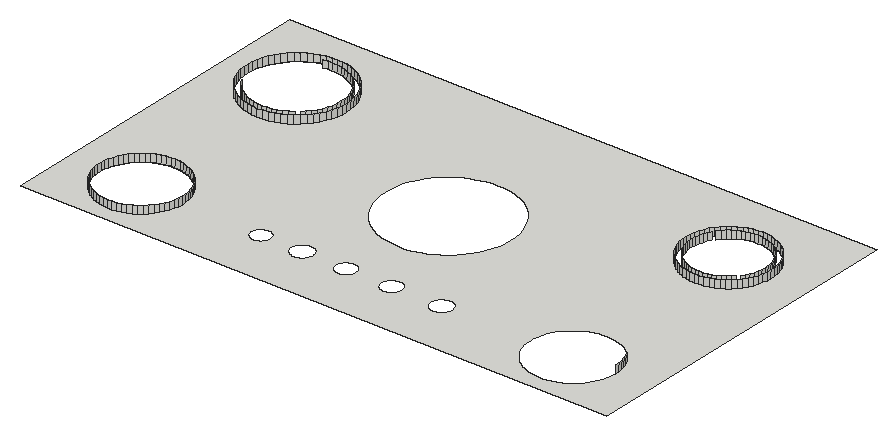
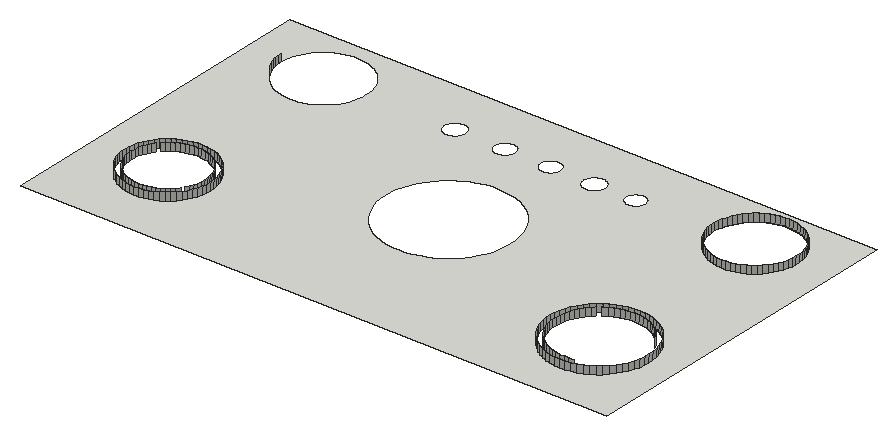
# SketchUp Ruby script. Lengths in inches.
U = 1.inch
M = Sketchup.active_model
def pt(a) = Geom::Point3d.new(a.map { |v| v * U })
def face(e, loops, mat)
  f = e.add_face(loops[0].map { |a| pt(a) })
  loops[1..].each { |l| e.add_face(l.map { |a| pt(a) }).erase! }
  f.material = f.back_material = mat if mat
  f
end
# faces: each face lists its corners as indices into pts; further lists are holes
def faces(e, pts, list, mat = nil) = list.each { |f| face(e, (f[0].is_a?(Array) ? f : [f]).map { |l| l.map { |i| pts[i] } }, mat) }
# xy, xz, yz: faces in a plane at the given z, y or x. An outline is a flat list of corners, or four numbers for a rectangle; further outlines are holes
def ring(l) = l.size == 4 ? [[l[0], l[1]], [l[2], l[1]], [l[2], l[3]], [l[0], l[3]]] : l.each_slice(2).to_a
def flat(e, list, mat, &to3) = list.each { |f| face(e, (f[0].is_a?(Array) ? f : [f]).map { |l| ring(l).map { |u, v| to3.(u, v) } }, mat) }
def xy(e, z, list, mat = nil) = flat(e, list, mat) { |x, y| [x, y, z] }
def xz(e, y, list, mat = nil) = flat(e, list, mat) { |x, z| [x, y, z] }
def yz(e, x, list, mat = nil) = flat(e, list, mat) { |y, z| [x, y, z] }
def lines(e, pts, list) = list.each { |a, b| e.add_line(pt(pts[a]), pt(pts[b])) }
# prism: a flat outline (further loops are holes) pulled along v
def prism(e, loops, v, mat = nil)
  f = face(e, loops, mat); d = Geom::Vector3d.new(v.map { |x| x * U })
  f.pushpull(f.normal.samedirection?(d) ? d.length : -d.length)
end
def box(e, o, s, mat = nil) = prism(e, [[o, [o[0] + s[0], o[1], o[2]], [o[0] + s[0], o[1] + s[1], o[2]], [o[0], o[1] + s[1], o[2]]]], [0, 0, s[2]], mat)
def at(x, y, z, deg = 0) = Geom::Transformation.translation(pt([x, y, z])) * Geom::Transformation.rotation(ORIGIN, Z_AXIS, deg.degrees)
def axes(o, x, y, z) = Geom::Transformation.new([*x, 0, *y, 0, *z, 0, *pt(o).to_a, 1])
def part(name) = M.definitions.add(name)
# library, detail: a bought-in or finely detailed component or shape, given as its bounding box
def library(name, o, s) = part(name).tap { |d| box(d.entities, o, s) }
def detail(e, o, s) = box(e.add_group.entities, o, s)
def put(e, d, t, mat = nil) = e.add_instance(d, t).tap { |i| i.material = mat if mat }
def group(e, t, mat = nil) = e.add_group.tap { |g| g.transformation = t; g.material = mat if mat }.entities
root = M.entities
xy(root,253.1875,[[[597.55,622.78,883.3,786.9],[739.6875,675.19,736.49,675.36,733.32,675.86,730.22,676.69,727.23,677.84,724.375,679.29,721.6875,681.04,719.19,683.06,716.93,685.32,714.91,687.82,713.16,690.5,711.71,693.36,710.5625,696.35,709.73,699.45,709.23,702.61,709.0625,705.82,709.23,709.02,709.73,712.18,710.5625,715.28,711.71,718.27,713.16,721.13,714.91,723.82,716.93,726.31,719.19,728.57,721.6875,730.59,724.375,732.34,727.23,733.79,730.22,734.94,733.32,735.77,736.49,736.27,739.6875,736.44,742.89,736.27,746.05,735.77,749.15,734.94,752.14,733.79,755,732.34,757.6875,730.59,760.18,728.57,762.45,726.31,764.46,723.82,766.21,721.13,767.66,718.27,768.8125,715.28,769.64,712.18,770.14,709.02,770.3125,705.82,770.14,702.61,769.64,699.45,768.8125,696.35,767.66,693.36,766.21,690.5,764.46,687.82,762.45,685.32,760.18,683.06,757.6875,681.04,755,679.29,752.14,677.84,749.15,676.69,746.05,675.86,742.89,675.36],[634.71,720.65,632.18,720.78,629.67,721.18,627.22,721.84,624.85,722.74,622.58,723.9,620.46,725.28,618.48,726.875,616.6875,728.67,615.09,730.64,613.71,732.77,612.56,735.03,611.65,737.4,610.99,739.86,610.59,742.36,610.46,744.9,610.59,747.43,610.99,749.94,611.65,752.39,612.56,754.76,613.71,757.02,615.09,759.15,616.6875,761.125,618.48,762.92,620.46,764.52,622.58,765.9,624.85,767.05,627.22,767.96,629.67,768.62,632.18,769.02,634.71,769.15,637.24,769.02,639.75,768.62,642.2,767.96,644.57,767.05,646.83,765.9,648.96,764.52,650.9375,762.92,652.73,761.125,654.33,759.15,655.71,757.02,656.86,754.76,657.77,752.39,658.43,749.94,658.83,747.43,658.96,744.9,658.83,742.36,658.43,739.86,657.77,737.4,656.86,735.03,655.71,732.77,654.33,730.64,652.73,728.67,650.9375,726.875,648.96,725.28,646.83,723.9,644.57,722.74,642.2,721.84,639.75,721.18,637.24,720.78],[844.95,724.15,842.78,724.26,840.64,724.6,838.54,725.16,836.51,725.94,834.58,726.93,832.76,728.11,831.07,729.48,829.53,731.01,828.16,732.7,826.98,734.52,826,736.46,825.22,738.49,824.66,740.58,824.32,742.73,824.2,744.9,824.32,747.07,824.66,749.21,825.22,751.31,826,753.34,826.98,755.27,828.16,757.09,829.53,758.78,831.07,760.32,832.76,761.69,834.58,762.87,836.51,763.85,838.54,764.63,840.64,765.19,842.78,765.53,844.95,765.65,847.12,765.53,849.27,765.19,851.36,764.63,853.39,763.85,855.33,762.87,857.15,761.69,858.84,760.32,860.37,758.78,861.74,757.09,862.92,755.27,863.91,753.34,864.6875,751.31,865.25,749.21,865.59,747.07,865.7,744.9,865.59,742.73,865.25,740.58,864.6875,738.49,863.91,736.46,862.92,734.52,861.74,732.7,860.37,731.01,858.84,729.48,857.15,728.11,855.33,726.93,853.39,725.94,851.36,725.16,849.27,724.6,847.12,724.26],[844.95,629.31,842.78,629.42,840.64,629.76,838.54,630.32,836.51,631.1,834.58,632.09,832.76,633.27,831.07,634.64,829.53,636.17,828.16,637.86,826.98,639.68,826,641.62,825.22,643.65,824.66,645.74,824.32,647.89,824.2,650.06,824.32,652.23,824.66,654.375,825.22,656.47,826,658.5,826.98,660.43,828.16,662.26,829.53,663.94,831.07,665.48,832.76,666.85,834.58,668.03,836.51,669.02,838.54,669.79,840.64,670.36,842.78,670.7,844.95,670.81,847.12,670.7,849.27,670.36,851.36,669.79,853.39,669.02,855.33,668.03,857.15,666.85,858.84,665.48,860.37,663.94,861.74,662.26,862.92,660.43,863.91,658.5,864.6875,656.47,865.25,654.375,865.59,652.23,865.7,650.06,865.59,647.89,865.25,645.74,864.6875,643.65,863.91,641.62,862.92,639.68,861.74,637.86,860.37,636.17,858.84,634.64,857.15,633.27,855.33,632.09,853.39,631.1,851.36,630.32,849.27,629.76,847.12,629.42],[634.4,629.8125,632.28,629.96,630.19,630.32,628.15,630.9,626.1875,631.69,624.3125,632.68,622.55,633.86,620.93,635.22,619.45,636.74,618.14,638.41,617.02,640.21,616.08,642.11,615.36,644.1,614.84,646.16,614.54,648.26,614.46,650.375,614.61,652.49,614.97,654.58,615.55,656.61,616.34,658.58,617.33,660.45,618.51,662.21,619.875,663.84,621.4,665.32,623.0625,666.625,624.86,667.75,626.76,668.68,628.75,669.41,630.81,669.93,632.91,670.23,635.02,670.31,637.14,670.16,639.23,669.8,641.27,669.22,643.23,668.43,645.11,667.4375,646.87,666.25,648.49,664.9,649.97,663.375,651.28,661.71,652.4,659.91,653.33,658.01,654.0625,656.02,654.58,653.96,654.88,651.86,654.96,649.74,654.8125,647.63,654.45,645.54,653.87,643.5,653.08,641.54,652.09,639.66,650.91,637.9,649.55,636.28,648.02,634.8,646.36,633.49,644.5625,632.37,642.66,631.43,640.67,630.71,638.61,630.1875,636.51,629.89],[713.34,644.32,712.77,644.35,712.21,644.4375,711.66,644.58,711.125,644.79,710.62,645.05,710.14,645.36,709.7,645.71,709.3,646.12,708.9375,646.56,708.63,647.04,708.37,647.54,708.17,648.07,708.02,648.625,707.93,649.1875,707.9,649.75,707.93,650.32,708.02,650.89,708.17,651.43,708.37,651.97,708.63,652.47,708.9375,652.95,709.3,653.39,709.7,653.8,710.14,654.15,710.62,654.46,711.125,654.72,711.66,654.93,712.21,655.07,712.77,655.16,713.34,655.19,713.91,655.16,714.47,655.07,715.02,654.93,715.55,654.72,716.06,654.46,716.53,654.15,716.98,653.8,717.38,653.39,717.74,652.95,718.05,652.47,718.31,651.97,718.51,651.43,718.66,650.89,718.75,650.32,718.78,649.75,718.75,649.1875,718.66,648.625,718.51,648.07,718.31,647.54,718.05,647.04,717.74,646.56,717.38,646.12,716.98,645.71,716.53,645.36,716.06,645.05,715.55,644.79,715.02,644.58,714.47,644.4375,713.91,644.35],[781.2,644.44,780.65,644.47,780.1,644.56,779.5625,644.7,779.04,644.9,778.55,645.15,778.08,645.46,777.65,645.81,777.26,646.2,776.91,646.63,776.6,647.1,776.35,647.59,776.15,648.11,776.01,648.65,775.92,649.2,775.89,649.75,775.92,650.31,776.01,650.86,776.15,651.4,776.35,651.92,776.6,652.41,776.91,652.88,777.26,653.31,777.65,653.7,778.08,654.05,778.55,654.36,779.04,654.61,779.5625,654.81,780.1,654.95,780.65,655.04,781.2,655.07,781.76,655.04,782.31,654.95,782.85,654.81,783.36,654.61,783.86,654.36,784.33,654.05,784.76,653.7,785.15,653.31,785.5,652.88,785.8,652.41,786.06,651.92,786.26,651.4,786.4,650.86,786.49,650.31,786.52,649.75,786.49,649.2,786.4,648.65,786.26,648.11,786.06,647.59,785.8,647.1,785.5,646.63,785.15,646.2,784.76,645.81,784.33,645.46,783.86,645.15,783.36,644.9,782.85,644.7,782.31,644.56,781.76,644.47],[756.84,644.69,756.3125,644.72,755.79,644.8,755.28,644.94,754.78,645.13,754.31,645.37,753.86,645.66,753.45,645.99,753.08,646.37,752.74,646.78,752.46,647.22,752.21,647.7,752.02,648.19,751.89,648.7,751.8,649.23,751.78,649.75,751.8,650.28,751.89,650.81,752.02,651.32,752.21,651.8125,752.46,652.29,752.74,652.73,753.08,653.14,753.45,653.52,753.86,653.85,754.31,654.14,754.78,654.38,755.28,654.57,755.79,654.71,756.3125,654.79,756.84,654.82,757.37,654.79,757.89,654.71,758.4,654.57,758.9,654.38,759.37,654.14,759.82,653.85,760.23,653.52,760.6,653.14,760.94,652.73,761.22,652.29,761.46,651.8125,761.65,651.32,761.79,650.81,761.875,650.28,761.9,649.75,761.875,649.23,761.79,648.7,761.65,648.19,761.46,647.7,761.22,647.22,760.94,646.78,760.6,646.37,760.23,645.99,759.82,645.66,759.37,645.37,758.9,645.13,758.4,644.94,757.89,644.8,757.37,644.72],[734.71,644.78,734.19,644.81,733.68,644.89,733.18,645.03,732.69,645.21,732.23,645.45,731.79,645.73,731.39,646.06,731.02,646.43,730.69,646.83,730.41,647.27,730.17,647.73,729.98,648.22,729.85,648.72,729.77,649.23,729.74,649.75,729.77,650.27,729.85,650.79,729.98,651.29,730.17,651.78,730.41,652.24,730.69,652.68,731.02,653.08,731.39,653.45,731.79,653.78,732.23,654.0625,732.69,654.3,733.18,654.48,733.68,654.62,734.19,654.7,734.71,654.73,735.23,654.7,735.75,654.62,736.25,654.48,736.74,654.3,737.2,654.0625,737.64,653.78,738.04,653.45,738.41,653.08,738.74,652.68,739.02,652.24,739.26,651.78,739.44,651.29,739.58,650.79,739.66,650.27,739.6875,649.75,739.66,649.23,739.58,648.72,739.44,648.22,739.26,647.73,739.02,647.27,738.74,646.83,738.41,646.43,738.04,646.06,737.64,645.73,737.2,645.45,736.74,645.21,736.25,645.03,735.75,644.89,735.23,644.81],[693.15,644.94,692.64,644.97,692.14,645.05,691.66,645.18,691.1875,645.36,690.74,645.59,690.32,645.86,689.93,646.18,689.57,646.53,689.25,646.93,688.98,647.35,688.75,647.8,688.57,648.27,688.4375,648.75,688.36,649.25,688.33,649.75,688.36,650.26,688.4375,650.76,688.57,651.24,688.75,651.71,688.98,652.16,689.25,652.58,689.57,652.97,689.93,653.33,690.32,653.65,690.74,653.92,691.1875,654.15,691.66,654.33,692.14,654.46,692.64,654.54,693.15,654.57,693.65,654.54,694.15,654.46,694.63,654.33,695.1,654.15,695.55,653.92,695.97,653.65,696.37,653.33,696.72,652.97,697.04,652.58,697.3125,652.16,697.54,651.71,697.72,651.24,697.85,650.76,697.93,650.26,697.96,649.75,697.93,649.25,697.85,648.75,697.72,648.27,697.54,647.8,697.3125,647.35,697.04,646.93,696.72,646.53,696.37,646.18,695.97,645.86,695.55,645.59,695.1,645.36,694.63,645.18,694.15,645.05,693.65,644.97]]])
p = [[632.28,629.96,253.1875],[634.4,629.8125,253.1875],[634.4,629.8125,256.875],[632.28,629.96,256.875],[636.51,629.89,253.1875],[636.51,629.89,256.875],
  [638.61,630.1875,253.1875],[638.61,630.1875,256.875],[630.19,630.32,253.1875],[630.19,630.32,256.875],[640.67,630.71,253.1875],[640.67,630.71,256.875],
  [628.15,630.9,253.1875],[628.15,630.9,256.875],[642.66,631.43,253.1875],[642.66,631.43,256.875],[626.1875,631.69,253.1875],[626.1875,631.69,256.875],
  [644.5625,632.37,253.1875],[644.5625,632.37,256.875],[624.3125,632.68,253.1875],[624.3125,632.68,256.875],[646.36,633.49,253.1875],[646.36,633.49,256.875],
  [622.55,633.86,253.1875],[622.55,633.86,256.875],[648.02,634.8,253.1875],[648.02,634.8,256.875],[620.93,635.22,253.1875],[620.93,635.22,256.875],
  [649.55,636.28,253.1875],[649.55,636.28,256.875],[619.45,636.74,253.1875],[619.45,636.74,256.875],[650.91,637.9,253.1875],[650.91,637.9,256.875],
  [618.14,638.41,253.1875],[618.14,638.41,256.875],[652.09,639.66,253.1875],[652.09,639.66,256.875],[617.02,640.21,253.1875],[617.02,640.21,256.875],
  [653.08,641.54,253.1875],[653.08,641.54,256.875],[616.08,642.11,253.1875],[616.08,642.11,256.875],[653.87,643.5,253.1875],[653.87,643.5,256.875],
  [615.36,644.1,253.1875],[615.36,644.1,256.875],[654.45,645.54,253.1875],[654.45,645.54,256.875],[614.84,646.16,253.1875],[614.84,646.16,256.875],
  [654.8125,647.63,253.1875],[654.8125,647.63,256.875],[614.54,648.26,253.1875],[614.54,648.26,256.875],[654.96,649.74,253.1875],[654.96,649.74,256.875],
  [614.46,650.375,253.1875],[614.46,650.375,256.875],[654.88,651.86,253.1875],[654.88,651.86,256.875],[865.7,650.06,253.1875],[865.59,652.23,253.1875],
  [865.59,652.23,256.875],[865.7,650.06,256.875],[614.61,652.49,253.1875],[614.61,652.49,256.875],[654.58,653.96,253.1875],[654.58,653.96,256.875],
  [865.25,654.375,253.1875],[865.25,654.375,256.875],[614.97,654.58,253.1875],[614.97,654.58,256.875],[654.0625,656.02,253.1875],[654.0625,656.02,256.875],
  [864.6875,656.47,253.1875],[864.6875,656.47,256.875],[615.55,656.61,253.1875],[615.55,656.61,256.875],[653.33,658.01,253.1875],[653.33,658.01,256.875],
  [863.91,658.5,253.1875],[863.91,658.5,256.875],[616.34,658.58,253.1875],[616.34,658.58,256.875],[652.4,659.91,253.1875],[652.4,659.91,256.875],
  [862.92,660.43,253.1875],[862.92,660.43,256.875],[617.33,660.45,253.1875],[617.33,660.45,256.875],[651.28,661.71,253.1875],[651.28,661.71,256.875],
  [618.51,662.21,253.1875],[618.51,662.21,256.875],[649.97,663.375,253.1875],[649.97,663.375,256.875],[619.875,663.84,253.1875],[619.875,663.84,256.875],
  [648.49,664.9,253.1875],[648.49,664.9,256.875],[621.4,665.32,253.1875],[621.4,665.32,256.875],[646.87,666.25,253.1875],[646.87,666.25,256.875],
  [623.0625,666.625,253.1875],[623.0625,666.625,256.875],[645.11,667.4375,253.1875],[645.11,667.4375,256.875],[624.86,667.75,253.1875],[624.86,667.75,256.875],
  [643.23,668.43,253.1875],[643.23,668.43,256.875],[626.76,668.68,253.1875],[626.76,668.68,256.875],[641.27,669.22,253.1875],[641.27,669.22,256.875],
  [628.75,669.41,253.1875],[628.75,669.41,256.875],[639.23,669.8,253.1875],[639.23,669.8,256.875],[630.81,669.93,253.1875],[630.81,669.93,256.875],
  [637.14,670.16,253.1875],[637.14,670.16,256.875],[632.91,670.23,253.1875],[632.91,670.23,256.875],[635.02,670.31,253.1875],[635.02,670.31,256.875],
  [632.18,720.78,253.1875],[634.71,720.65,253.1875],[634.71,720.65,256.875],[632.18,720.78,256.875],[637.24,720.78,253.1875],[637.24,720.78,256.875],
  [629.67,721.18,253.1875],[629.67,721.18,256.875],[639.75,721.18,253.1875],[639.75,721.18,256.875],[627.22,721.84,253.1875],[627.22,721.84,256.875],
  [642.2,721.84,253.1875],[642.2,721.84,256.875],[624.85,722.74,253.1875],[624.85,722.74,256.875],[644.57,722.74,253.1875],[644.57,722.74,256.875],
  [622.58,723.9,253.1875],[622.58,723.9,256.875],[646.83,723.9,253.1875],[646.83,723.9,256.875],[634.71,723.48,253.1875],[632.47,723.59,253.1875],
  [632.47,723.59,256.875],[634.71,723.48,256.875],[636.95,723.59,253.1875],[636.95,723.59,256.875],[630.26,723.94,253.1875],[630.26,723.94,256.875],
  [639.16,723.94,253.1875],[639.16,723.94,256.875],[620.46,725.28,253.1875],[620.46,725.28,256.875],[628.09,724.53,253.1875],[628.09,724.53,256.875],
  [641.33,724.53,253.1875],[641.33,724.53,256.875],[648.96,725.28,253.1875],[648.96,725.28,256.875],[842.78,724.26,253.1875],[844.95,724.15,253.1875],
  [844.95,724.15,256.875],[842.78,724.26,256.875],[847.12,724.26,253.1875],[847.12,724.26,256.875],[840.64,724.6,253.1875],[840.64,724.6,256.875],
  [849.27,724.6,253.1875],[849.27,724.6,256.875],[626,725.33,253.1875],[626,725.33,256.875],[643.42,725.33,253.1875],[643.42,725.33,256.875],
  [838.54,725.16,253.1875],[838.54,725.16,256.875],[851.36,725.16,253.1875],[851.36,725.16,256.875],[836.51,725.94,253.1875],[836.51,725.94,256.875],
  [853.39,725.94,253.1875],[853.39,725.94,256.875],[618.48,726.875,253.1875],[618.48,726.875,256.875],[624,726.35,253.1875],[624,726.35,256.875],
  [645.42,726.35,253.1875],[645.42,726.35,256.875],[650.9375,726.875,253.1875],[650.9375,726.875,256.875],[834.58,726.93,253.1875],[834.58,726.93,256.875],
  [855.33,726.93,253.1875],[855.33,726.93,256.875],[622.12,727.57,253.1875],[622.12,727.57,256.875],[647.3,727.57,253.1875],[647.3,727.57,256.875],
  [647.3,727.57,255.1875],[616.6875,728.67,253.1875],[616.6875,728.67,256.875],[652.73,728.67,253.1875],[652.73,728.67,256.875],[832.76,728.11,253.1875],
  [832.76,728.11,256.875],[857.15,728.11,253.1875],[857.15,728.11,256.875],[844.95,726.98,253.1875],[843.08,727.07,253.1875],[843.08,727.07,256.875],
  [844.95,726.98,256.875],[846.82,727.07,253.1875],[846.82,727.07,256.875],[841.23,727.37,253.1875],[841.23,727.37,256.875],[848.68,727.37,253.1875],
  [848.68,727.37,256.875],[839.41,727.85,253.1875],[839.41,727.85,256.875],[850.49,727.85,253.1875],[850.49,727.85,256.875],[620.375,728.98,253.1875],
  [620.375,728.98,256.875],[837.66,728.53,253.1875],[837.66,728.53,256.875],[852.24,728.53,253.1875],[852.24,728.53,256.875],[831.07,729.48,253.1875],
  [831.07,729.48,256.875],[858.84,729.48,253.1875],[858.84,729.48,256.875],[835.99,729.38,253.1875],[835.99,729.38,256.875],[853.91,729.38,253.1875],
  [853.91,729.38,256.875],[615.09,730.64,253.1875],[615.09,730.64,256.875],[654.33,730.64,253.1875],[654.33,730.64,256.875],[619.69,729.66,253.1875],
  [619.69,729.66,255.1875],[618.79,730.5625,255.1875],[618.79,730.5625,256.875],[650.63,730.5625,253.1875],[649.04,728.98,253.1875],[649.04,728.98,255.1875],
  [649.04,728.98,256.875],[650.63,730.5625,256.875],[834.42,730.4,253.1875],[834.42,730.4,254.5],[834.42,730.4,256.875],[855.49,730.4,253.1875],
  [855.49,730.4,256.875],[829.53,731.01,253.1875],[829.53,731.01,256.875],[860.37,731.01,253.1875],[860.37,731.01,256.875],[856.94,731.58,253.1875],
  [856.94,731.58,256.875],[613.71,732.77,253.1875],[613.71,732.77,256.875],[618.09,731.4375,255.1875],[618.09,731.4375,253.1875],[617.38,732.31,253.1875],
  [617.38,732.31,256.875],[652.04,732.31,253.1875],[652.04,732.31,256.875],[655.71,732.77,253.1875],[655.71,732.77,256.875],[828.16,732.7,253.1875],
  [828.16,732.7,256.875],[861.74,732.7,253.1875],[861.74,732.7,256.875],[832.96,731.58,253.1875],[831.63,732.91,253.1875],[831.63,732.91,256.875],
  [832.96,731.58,256.875],[832.96,731.58,254.5],[858.27,732.91,253.1875],[858.27,732.91,256.875],[858.27,732.91,254.5],[616.16,734.1875,253.1875],
  [616.16,734.1875,256.875],[653.26,734.1875,253.1875],[653.26,734.1875,256.875],[826.98,734.52,253.1875],[826.98,734.52,256.875],[862.92,734.52,253.1875],
  [862.92,734.52,256.875],[612.56,735.03,253.1875],[612.56,735.03,256.875],[656.86,735.03,253.1875],[656.86,735.03,256.875],[830.45,734.36,253.1875],
  [830.45,734.36,256.875],[654.28,736.19,253.1875],[654.28,736.19,256.875],[829.43,735.9375,253.1875],[829.43,735.9375,256.875],[860.47,735.9375,253.1875],
  [859.45,734.36,253.1875],[859.45,734.36,254.5],[859.45,734.36,256.875],[860.47,735.9375,256.875],[826,736.46,253.1875],[826,736.46,256.875],
  [863.91,736.46,253.1875],[863.91,736.46,256.875],[611.65,737.4,253.1875],[611.65,737.4,256.875],[657.77,737.4,253.1875],[657.77,737.4,256.875],
  [828.58,737.61,253.1875],[828.58,737.61,256.875],[861.32,737.61,253.1875],[861.32,737.61,256.875],[655.08,738.28,253.1875],[655.08,738.28,256.875],
  [825.22,738.49,253.1875],[825.22,738.49,256.875],[864.6875,738.49,253.1875],[864.6875,738.49,256.875],[610.99,739.86,253.1875],[610.99,739.86,256.875],
  [658.43,739.86,253.1875],[658.43,739.86,256.875],[827.91,739.36,253.1875],[827.91,739.36,256.875],[862,739.36,253.1875],[862,739.36,256.875],
  [655.66,740.44,253.1875],[655.66,740.44,256.875],[824.66,740.58,253.1875],[824.66,740.58,256.875],[865.25,740.58,253.1875],[865.25,740.58,256.875],
  [827.42,741.17,253.1875],[827.42,741.17,256.875],[862.48,741.17,253.1875],[862.48,741.17,256.875],[610.59,742.36,253.1875],[610.59,742.36,256.875],
  [658.83,742.36,253.1875],[658.83,742.36,256.875],[656.01,742.66,253.1875],[656.01,742.66,256.875],[824.32,742.73,253.1875],[824.32,742.73,256.875],
  [865.59,742.73,253.1875],[865.59,742.73,256.875],[827.13,743.02,253.1875],[827.13,743.02,256.875],[862.77,743.02,253.1875],[862.77,743.02,256.875],
  [610.46,744.9,253.1875],[610.46,744.9,256.875],[658.96,744.9,253.1875],[658.96,744.9,256.875],[656.13,744.9,253.1875],[656.13,744.9,256.875],
  [824.2,744.9,253.1875],[824.2,744.9,256.875],[865.7,744.9,253.1875],[865.7,744.9,256.875],[827.03,744.9,253.1875],[827.03,744.9,256.875],
  [862.875,744.9,253.1875],[862.875,744.9,256.875],[610.59,747.43,253.1875],[610.59,747.43,256.875],[656.01,747.14,253.1875],[656.01,747.14,256.875],
  [658.83,747.43,253.1875],[658.83,747.43,256.875],[824.32,747.07,253.1875],[824.32,747.07,256.875],[827.13,746.77,253.1875],[827.13,746.77,256.875],
  [862.77,746.77,253.1875],[862.77,746.77,256.875],[865.59,747.07,253.1875],[865.59,747.07,256.875],[827.42,748.625,253.1875],[827.42,748.625,256.875],
  [862.48,748.625,253.1875],[862.48,748.625,256.875],[655.66,749.35,253.1875],[655.66,749.35,256.875],[824.66,749.21,253.1875],[824.66,749.21,256.875],
  [865.25,749.21,253.1875],[865.25,749.21,256.875],[610.99,749.94,253.1875],[610.99,749.94,256.875],[658.43,749.94,253.1875],[658.43,749.94,256.875],
  [827.91,750.4375,253.1875],[827.91,750.4375,256.875],[862,750.4375,253.1875],[862,750.4375,256.875],[825.22,751.31,253.1875],[825.22,751.31,256.875],
  [864.6875,751.31,253.1875],[864.6875,751.31,256.875],[655.08,751.52,253.1875],[655.08,751.52,256.875],[611.65,752.39,253.1875],[611.65,752.39,256.875],
  [657.77,752.39,253.1875],[657.77,752.39,256.875],[828.58,752.1875,253.1875],[828.58,752.1875,256.875],[861.32,752.1875,253.1875],[861.32,752.1875,256.875],
  [826,753.34,253.1875],[826,753.34,256.875],[863.91,753.34,253.1875],[863.91,753.34,256.875],[654.28,753.61,253.1875],[654.28,753.61,256.875],
  [829.43,753.86,253.1875],[829.43,753.86,254.5],[829.43,753.86,256.875],[860.47,753.86,253.1875],[860.47,753.86,256.875],[612.56,754.76,253.1875],
  [612.56,754.76,256.875],[656.86,754.76,253.1875],[656.86,754.76,256.875],[826.98,755.27,253.1875],[826.98,755.27,256.875],[862.92,755.27,253.1875],
  [862.92,755.27,256.875],[653.26,755.61,253.1875],[653.26,755.61,256.875],[859.45,755.43,253.1875],[859.45,755.43,256.875],[613.71,757.02,253.1875],
  [613.71,757.02,256.875],[655.71,757.02,253.1875],[655.71,757.02,256.875],[828.16,757.09,253.1875],[828.16,757.09,256.875],[861.74,757.09,253.1875],
  [861.74,757.09,256.875],[830.45,755.43,253.1875],[831.63,756.89,253.1875],[831.63,756.89,256.875],[830.45,755.43,256.875],[830.45,755.43,254.5],
  [858.27,756.89,253.1875],[858.27,756.89,256.875],[858.27,756.89,254.5],[652.04,757.49,253.1875],[652.04,757.49,256.875],[652.04,757.49,255.1875],
  [832.96,758.22,253.1875],[832.96,758.22,256.875],[615.09,759.15,253.1875],[615.09,759.15,256.875],[654.33,759.15,253.1875],[654.33,759.15,256.875],
  [829.53,758.78,253.1875],[829.53,758.78,256.875],[860.37,758.78,253.1875],[860.37,758.78,256.875],[834.42,759.4,253.1875],[834.42,759.4,256.875],
  [855.49,759.4,253.1875],[856.94,758.22,253.1875],[856.94,758.22,254.5],[856.94,758.22,256.875],[855.49,759.4,256.875],[831.07,760.32,253.1875],
  [831.07,760.32,256.875],[858.84,760.32,253.1875],[858.84,760.32,256.875],[616.6875,761.125,253.1875],[616.6875,761.125,256.875],[649.04,760.82,253.1875],
  [650.63,759.23,253.1875],[650.63,759.23,255.1875],[650.63,759.23,256.875],[649.04,760.82,256.875],[652.73,761.125,253.1875],[652.73,761.125,256.875],
  [835.99,760.42,253.1875],[835.99,760.42,256.875],[853.91,760.42,253.1875],[853.91,760.42,256.875],[832.76,761.69,253.1875],[832.76,761.69,256.875],
  [857.15,761.69,253.1875],[857.15,761.69,256.875],[837.66,761.27,253.1875],[837.66,761.27,256.875],[852.24,761.27,253.1875],[852.24,761.27,256.875],
  [647.3,762.23,253.1875],[647.3,762.23,256.875],[618.48,762.92,253.1875],[618.48,762.92,256.875],[650.9375,762.92,253.1875],[650.9375,762.92,256.875],
  [839.41,761.94,253.1875],[839.41,761.94,256.875],[850.49,761.94,253.1875],[850.49,761.94,256.875],[834.58,762.87,253.1875],[834.58,762.87,256.875],
  [855.33,762.87,253.1875],[855.33,762.87,256.875],[841.23,762.43,253.1875],[841.23,762.43,256.875],[848.68,762.43,253.1875],[848.68,762.43,256.875],
  [645.42,763.45,253.1875],[645.42,763.45,256.875],[843.08,762.72,253.1875],[843.08,762.72,256.875],[846.82,762.72,253.1875],[846.82,762.72,256.875],
  [844.95,762.82,253.1875],[844.95,762.82,256.875],[620.46,764.52,253.1875],[620.46,764.52,256.875],[648.96,764.52,253.1875],[648.96,764.52,256.875],
  [836.51,763.85,253.1875],[836.51,763.85,256.875],[853.39,763.85,253.1875],[853.39,763.85,256.875],[643.42,764.47,253.1875],[643.42,764.47,256.875],
  [838.54,764.63,253.1875],[838.54,764.63,256.875],[851.36,764.63,253.1875],[851.36,764.63,256.875],[622.58,765.9,253.1875],[622.58,765.9,256.875],
  [641.33,765.27,253.1875],[641.33,765.27,256.875],[646.83,765.9,253.1875],[646.83,765.9,256.875],[840.64,765.19,253.1875],[840.64,765.19,256.875],
  [849.27,765.19,253.1875],[849.27,765.19,256.875],[842.78,765.53,253.1875],[842.78,765.53,256.875],[847.12,765.53,253.1875],[847.12,765.53,256.875],
  [639.16,765.85,253.1875],[639.16,765.85,256.875],[844.95,765.65,253.1875],[844.95,765.65,256.875],[624.85,767.05,253.1875],[624.85,767.05,256.875],
  [630.26,765.85,253.1875],[632.47,766.2,253.1875],[632.47,766.2,256.875],[630.26,765.85,256.875],[636.95,766.2,253.1875],[636.95,766.2,256.875],
  [644.57,767.05,253.1875],[644.57,767.05,256.875],[634.71,766.32,253.1875],[634.71,766.32,256.875],[627.22,767.96,253.1875],[627.22,767.96,256.875],
  [642.2,767.96,253.1875],[642.2,767.96,256.875],[629.67,768.62,253.1875],[629.67,768.62,256.875],[639.75,768.62,253.1875],[639.75,768.62,256.875],
  [632.18,769.02,253.1875],[632.18,769.02,256.875],[637.24,769.02,253.1875],[637.24,769.02,256.875],[634.71,769.15,253.1875],[634.71,769.15,256.875]]
faces(root,p,[[0,1,2,3],[1,4,5,2],[4,6,7,5],[8,0,3,9],[6,10,11,7],[12,8,9,13],[10,14,15,11],[16,12,13,17],
  [14,18,19,15],[20,16,17,21],[18,22,23,19],[24,20,21,25],[22,26,27,23],[28,24,25,29],[26,30,31,27],[32,28,29,33],
  [30,34,35,31],[36,32,33,37],[34,38,39,35],[40,36,37,41],[38,42,43,39],[44,40,41,45],[42,46,47,43],[48,44,45,49],
  [46,50,51,47],[52,48,49,53],[50,54,55,51],[56,52,53,57],[54,58,59,55],[60,56,57,61],[58,62,63,59],[64,65,66,67],
  [68,60,61,69],[62,70,71,63],[65,72,73,66],[74,68,69,75],[70,76,77,71],[72,78,79,73],[80,74,75,81],[76,82,83,77],
  [78,84,85,79],[86,80,81,87],[82,88,89,83],[84,90,91,85],[92,86,87,93],[88,94,95,89],[96,92,93,97],[94,98,99,95],
  [100,96,97,101],[98,102,103,99],[104,100,101,105],[102,106,107,103],[108,104,105,109],[106,110,111,107],[112,108,109,113],[110,114,115,111],
  [116,112,113,117],[114,118,119,115],[120,116,117,121],[118,122,123,119],[124,120,121,125],[122,126,127,123],[128,124,125,129],[130,128,129,131],
  [126,130,131,127],[132,133,134,135],[133,136,137,134],[138,132,135,139],[136,140,141,137],[142,138,139,143],[140,144,145,141],[146,142,143,147],
  [144,148,149,145],[150,146,147,151],[148,152,153,149],[154,155,156,157],[158,154,157,159],[155,160,161,156],[162,158,159,163],[164,150,151,165],
  [160,166,167,161],[168,162,163,169],[152,170,171,153],[172,173,174,175],[173,176,177,174],[178,172,175,179],[176,180,181,177],[166,182,183,167],
  [184,168,169,185],[186,178,179,187],[180,188,189,181],[190,186,187,191],[188,192,193,189],[194,164,165,195],[182,196,197,183],[198,184,185,199],
  [170,200,201,171],[202,190,191,203],[192,204,205,193],[196,206,207,197],[208,198,199,209,210],[211,194,195,212],[200,213,214,201],[215,202,203,216],
  [204,217,218,205],[219,220,221,222],[223,219,222,224],[220,225,226,221],[227,223,224,228],[225,229,230,226],[231,227,228,232],[206,233,234,207],
  [229,235,236,230],[237,231,232,238],[239,215,216,240],[217,241,242,218],[235,243,244,236],[245,237,238,246],[247,211,212,248],[213,249,250,214],
  [233,251,252,253,254,234],[255,256,257,258,259],[243,260,261,262,244],[263,245,246,264],[265,239,240,266],[241,267,268,242],[269,263,264,270],[271,247,248,272],
  [254,253,273,274,275,276],[277,255,259,278],[249,279,280,250],[281,265,266,282],[267,283,284,268],[285,286,287,288,289],[290,269,270,291,292],[275,293,294,276],
  [295,277,278,296],[297,281,282,298],[283,299,300,284],[301,271,272,302],[279,303,304,280],[286,305,306,287],[307,295,296,308],[305,309,310,306],
  [311,312,313,314,315],[316,297,298,317],[299,318,319,300],[320,301,302,321],[303,322,323,304],[309,324,325,310],[326,311,315,327],[328,307,308,329],
  [330,316,317,331],[318,332,333,319],[334,320,321,335],[322,336,337,323],[324,338,339,325],[340,326,327,341],[342,328,329,343],[344,330,331,345],
  [332,346,347,333],[338,348,349,339],[350,340,341,351],[352,334,335,353],[336,354,355,337],[356,342,343,357],[358,344,345,359],[346,360,361,347],
  [348,362,363,349],[364,350,351,365],[366,352,353,367],[354,368,369,355],[370,356,357,371],[372,358,359,373],[360,374,375,361],[362,376,377,363],
  [378,364,365,379],[380,366,367,381],[382,370,371,383],[368,384,385,369],[386,372,373,387],[376,388,389,377],[390,378,379,391],[374,392,393,375],
  [388,394,395,389],[396,390,391,397],[398,382,383,399],[400,386,387,401],[392,402,403,393],[404,380,381,405],[384,406,407,385],[394,408,409,395],
  [410,396,397,411],[412,400,401,413],[402,414,415,403],[416,398,399,417],[418,404,405,419],[406,420,421,407],[408,422,423,409],[424,410,411,425],
  [426,412,413,427],[414,428,429,415],[430,416,417,431],[422,432,433,434,423],[435,424,425,436],[437,418,419,438],[420,439,440,421],[441,426,427,442],
  [428,443,444,429],[445,430,431,446],[447,435,436,448],[449,437,438,450],[439,451,452,440],[453,441,442,454],[443,455,456,444],[457,458,459,460,461],
  [462,447,448,463,464],[465,445,446,466,467],[458,468,469,459],[470,449,450,471],[451,472,473,452],[474,453,454,475],[455,476,477,456],[468,478,479,469],
  [480,481,482,483,484],[485,474,475,486],[476,487,488,477],[489,470,471,490],[491,492,493,494,495],[472,496,497,473],[478,498,499,479],[500,480,484,501],
  [502,485,486,503],[487,504,505,488],[498,506,507,499],[508,500,501,509],[510,491,495,511],[512,489,490,513],[496,514,515,497],[506,516,517,507],
  [518,508,509,519],[520,502,503,521],[504,522,523,505],[516,524,525,517],[526,518,519,527],[528,510,511,529],[524,530,531,525],[532,526,527,533],
  [530,534,535,531],[534,532,533,535],[536,512,513,537],[514,538,539,515],[540,520,521,541],[522,542,543,523],[544,528,529,545],[546,540,541,547],
  [542,548,549,543],[550,536,537,551],[552,544,545,553],[538,554,555,539],[556,546,547,557],[548,558,559,549],[560,556,557,561],[558,562,563,559],
  [564,552,553,565],[566,560,561,567],[562,566,567,563],[568,550,551,569],[570,571,572,573],[574,564,565,575],[554,576,577,555],[571,578,579,572],
  [578,574,575,579],[580,568,569,581],[576,582,583,577],[584,580,581,585],[582,586,587,583],[588,584,585,589],[586,590,591,587],[592,588,589,593],
  [590,592,593,591]])
